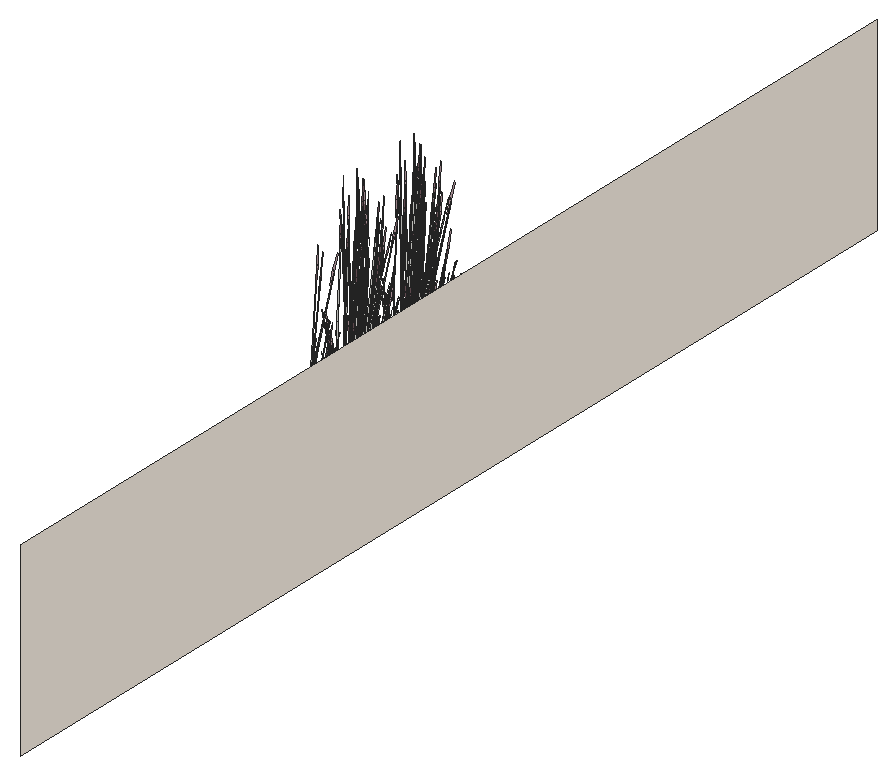
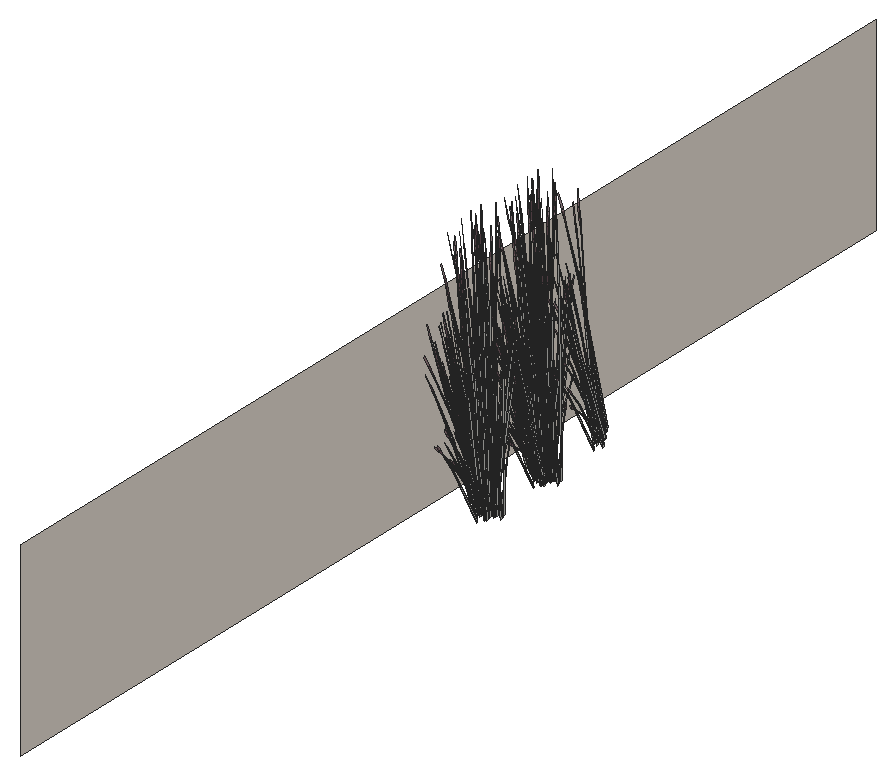
# SketchUp Ruby script. Lengths in inches.
U = 1.inch
M = Sketchup.active_model
def pt(a) = Geom::Point3d.new(a.map { |v| v * U })
def face(e, loops, mat)
  f = e.add_face(loops[0].map { |a| pt(a) })
  loops[1..].each { |l| e.add_face(l.map { |a| pt(a) }).erase! }
  f.material = f.back_material = mat if mat
  f
end
# faces: each face lists its corners as indices into pts; further lists are holes
def faces(e, pts, list, mat = nil) = list.each { |f| face(e, (f[0].is_a?(Array) ? f : [f]).map { |l| l.map { |i| pts[i] } }, mat) }
# xy, xz, yz: faces in a plane at the given z, y or x. An outline is a flat list of corners, or four numbers for a rectangle; further outlines are holes
def ring(l) = l.size == 4 ? [[l[0], l[1]], [l[2], l[1]], [l[2], l[3]], [l[0], l[3]]] : l.each_slice(2).to_a
def flat(e, list, mat, &to3) = list.each { |f| face(e, (f[0].is_a?(Array) ? f : [f]).map { |l| ring(l).map { |u, v| to3.(u, v) } }, mat) }
def xy(e, z, list, mat = nil) = flat(e, list, mat) { |x, y| [x, y, z] }
def xz(e, y, list, mat = nil) = flat(e, list, mat) { |x, z| [x, y, z] }
def yz(e, x, list, mat = nil) = flat(e, list, mat) { |y, z| [x, y, z] }
def lines(e, pts, list) = list.each { |a, b| e.add_line(pt(pts[a]), pt(pts[b])) }
# prism: a flat outline (further loops are holes) pulled along v
def prism(e, loops, v, mat = nil)
  f = face(e, loops, mat); d = Geom::Vector3d.new(v.map { |x| x * U })
  f.pushpull(f.normal.samedirection?(d) ? d.length : -d.length)
end
def box(e, o, s, mat = nil) = prism(e, [[o, [o[0] + s[0], o[1], o[2]], [o[0] + s[0], o[1] + s[1], o[2]], [o[0], o[1] + s[1], o[2]]]], [0, 0, s[2]], mat)
def at(x, y, z, deg = 0) = Geom::Transformation.translation(pt([x, y, z])) * Geom::Transformation.rotation(ORIGIN, Z_AXIS, deg.degrees)
def axes(o, x, y, z) = Geom::Transformation.new([*x, 0, *y, 0, *z, 0, *pt(o).to_a, 1])
def part(name) = M.definitions.add(name)
# library, detail: a bought-in or finely detailed component or shape, given as its bounding box
def library(name, o, s) = part(name).tap { |d| box(d.entities, o, s) }
def detail(e, o, s) = box(e.add_group.entities, o, s)
def put(e, d, t, mat = nil) = e.add_instance(d, t).tap { |i| i.material = mat if mat }
def group(e, t, mat = nil) = e.add_group.tap { |g| g.transformation = t; g.material = mat if mat }.entities
root = M.entities
M.materials.add("C01_Vanilla_Cream").color = [255, 246, 235]
M.materials.add("LightPink_Translucent").color = [144, 107, 117]
M.materials["LightPink_Translucent"].alpha = 0.75
c1 = part("blade")
p = [[2.15,0.21,22],[0,0.17,0],[0.09,0.45,0],[2.18,0.31,22],[2.29,0.31,22],[0.38,0.45,0],
  [2.48,0.24,33],[2.49,0.24,33],[2.48,0.22,33]]
faces(c1.entities,p,[[0,1,2,3],[4,5,2,3],[6,3,4,7],[8,0,3,6]])
c2 = part("seeds")
p = [[0.3,-0.1,1.38],[-0.01,-0.03,1.59],[-0.01,-0.03,0.03],[0.14,-0.07,-0.07],[0.29,-0.03,3],[0.15,0.01,3.11]]
faces(c2.entities,p,[[0,1,2,3],[1,0,4,5]],"LightPink_Translucent")
c3 = part("blade with seeds")
put(c3.entities,c1,at(0,0,0))
put(c3.entities,c2,axes([2.4,0.25,30.99],[1.5799,-0.05474,1.17369],[-0.12525,1.92788,0.29478],[-0.07173,-0.02425,1.56792]))
yz(root,354,[[30,654,234,690]],"C01_Vanilla_Cream")
put(root,c3,axes([342.72,109.8,658.14],[-0.07631,-0.33368,0.29039],[0.43626,-0.08811,-0.3749],[0.11718,0.09562,0.71734]))
put(root,c3,axes([344.36,108.77,655.65],[0,0.41426,-0.40713],[-0.55282,0,0],[0,0.09435,1.29153]))
put(root,c3,axes([342.97,108.82,657.18],[-0.18354,-0.07137,1.40529],[0.37983,-0.29943,0.11363],[0.23673,0.13508,0.60075]))
put(root,c3,axes([343.01,107.88,657.67],[-0.42697,-0.21524,1.13392],[0.45084,-0.33512,0.48925],[0.13776,0.20196,1.09604]))
put(root,c3,axes([343.65,109.63,656.27],[-0.27821,-0.11912,0.94186],[0.35924,-0.12103,0.69201],[0.09689,0.10252,0.20745]))
put(root,c3,axes([342.68,109.97,658.13],[0.29444,-0.35459,-0.09971],[0.4264,0.20428,-0.55346],[0.14822,0.10018,0.84097]))
put(root,c3,axes([342.29,110.27,657.86],[0.00146,-0.05015,1.45454],[0.42344,-0.22127,-0.13744],[0.14708,0.07898,0.2574]))
put(root,c3,axes([343.73,110.07,655.22],[0.036,-0.05981,1.44601],[0.45322,-0.17614,-0.2209],[0.1374,0.09116,0.2463]))
put(root,c3,axes([343.13,108.72,655.72],[0.18118,0.37929,-0.56754],[-0.52191,0.1366,-0.14895],[0.02003,0.12844,1.25274]))
put(root,c3,axes([343.03,109.8,657.84],[0.48758,-0.09847,-0.41901],[0.08529,0.37293,-0.32456],[0.13096,0.10687,0.80174]))
put(root,c3,axes([341.67,109.85,658.14],[0.14896,-0.31857,0.29039],[0.4346,0.09292,-0.3749],[0.03985,0.12826,0.71734]))
put(root,c3,axes([343.7,110.17,656.1875],[-0.31686,-0.01299,0.86149],[0.20925,-0.27594,0.47565],[0.12517,0.09804,0.67577]))
put(root,c3,axes([342.79,110.1,657.88],[-0.22457,0.26316,0.05273],[-0.3198,-0.15321,0.41509],[0.10339,0.08437,0.63295]))
put(root,c3,axes([342.26,110.99,658.63],[0.34145,-0.23766,-0.0532],[0.31287,0.26029,-0.24121],[0.02203,0.07375,0.7956]))
put(root,c3,axes([342.88,110.03,657.88],[-0.49145,0.09507,0.39362],[-0.08529,-0.37293,0.32456],[0.11558,0.10991,0.8145]))
put(root,c3,axes([342.66,109.51,656.125],[0.00872,-0.13732,1.17261],[0.41669,-0.15339,-0.25218],[0.12863,0.16436,0.50135]))
put(root,c3,axes([341.53,109.99,658.13],[0.48353,-0.19287,-0.09971],[0.23761,0.34232,-0.55346],[0.0638,0.14425,0.84097]))
put(root,c3,axes([341.94,109.97,657.84],[0.48573,0.10385,-0.41901],[-0.16649,0.35605,-0.32456],[0.04454,0.14335,0.80174]))
put(root,c3,axes([342.22,109.23,657.18],[-0.11295,-0.13301,1.40529],[0.52192,-0.11198,0.11363],[0.11796,0.20881,0.60075]))
put(root,c3,axes([341.77,109.9,658.08],[0.23583,0.33684,-0.58257],[-0.48546,0.18772,0.0703],[0.05515,0.16275,0.8241]))
put(root,c3,axes([341.41,110.75,657.87],[0.06263,0.06671,1.43454],[0.50546,0.02621,-0.22687],[0.05083,0.14712,0.11505]))
put(root,c3,axes([343.01,120.83,656.125],[-0.14045,0.08385,1.17261],[-0.42064,-0.14676,-0.25218],[0.07797,-0.18252,0.50135]))
put(root,c3,axes([343.35,121.45,658.08],[0.01286,-0.38319,-0.58257],[0.54141,0.02574,0.0703],[0.05714,-0.16234,0.8241]))
put(root,c3,axes([344.11,120.86,657.87],[-0.00477,-0.08245,1.43454],[-0.40285,-0.23829,-0.22687],[0.06228,-0.14445,0.11505]))
put(root,c3,axes([342.74,121.26,657.18],[-0.092,0.14239,1.40529],[-0.38596,-0.29467,0.11363],[0.17411,-0.18366,0.60075]))
put(root,c3,axes([344,120.56,657.86],[-0.05018,0.03164,1.45454],[-0.49165,-0.10676,-0.13744],[-0.0178,-0.13809,0.2574]))
put(root,c3,axes([342.49,120.17,656.27],[0.06339,0.24157,0.94186],[-0.35163,-0.13379,0.69201],[0.03784,-0.12369,0.20745]))
put(root,c3,axes([343.24,121.33,657.84],[-0.35372,-0.27835,-0.41901],[0.37366,-0.24377,-0.32456],[0.05382,-0.14142,0.80174]))
put(root,c3,axes([342.47,120.91,657.88],[0.48688,0.1083,0.39362],[-0.16649,0.35605,0.32456],[-0.02926,-0.14002,0.8145]))
put(root,c3,axes([343.61,121.47,658.13],[-0.54305,-0.02053,-0.09971],[0.01484,-0.38862,-0.55346],[0.03772,-0.14967,0.84097]))
put(root,c3,axes([343.57,121.22,657.71],[0.33433,-0.21811,-0.29039],[0.31649,0.24905,0.3749],[0.04815,-0.12654,0.71734]))
put(root,c3,axes([342.6,120.89,657.88],[0.36409,-0.14079,0.05273],[0.17821,0.25674,0.41509],[-0.03516,-0.11317,0.63295]))
put(root,c3,axes([343.99,121.09,655.22],[-0.07396,-0.03263,1.44601],[-0.18997,-0.3646,-0.2209],[0.12815,-0.09894,0.2463]))
put(root,c3,axes([343.57,121.31,657.88],[0.35185,0.28265,0.39362],[-0.37366,0.24377,0.32456],[0.0649,-0.13261,0.8145]))
put(root,c3,axes([343.7,121.34,657.88],[0.40605,0.0193,0.05273],[-0.01113,0.29147,0.41509],[0.04249,-0.11165,0.63295]))
put(root,c3,axes([343.4,121.53,658.14],[-0.33433,0.21811,0.29039],[-0.31649,-0.24905,-0.3749],[0.04815,-0.12654,0.71734]))
put(root,c3,axes([343.99,122.12,658.08],[0.2581,-0.32687,-0.58257],[0.45228,0.2323,0.0703],[0.15411,-0.11843,0.8241]))
put(root,c3,axes([341.2,121.17,655.95],[-0.30893,-0.41511,0],[0.51685,-0.2315,-0.42318],[0.11772,-0.05273,1.34243]))
put(root,c3,axes([343.98,121.97,657.84],[-0.12693,-0.37826,-0.41901],[0.48071,-0.06617,-0.32456],[0.13776,-0.1016,0.80174]))
put(root,c3,axes([344.2,122.24,658.13],[-0.45707,-0.22842,-0.09971],[0.26332,-0.3308,-0.55346],[0.12913,-0.11499,0.84097]))
put(root,c3,axes([341.62,121.1,655.65],[0.46245,-0.20713,-0.40713],[0.27641,0.37142,0],[0.10533,-0.04718,1.29153]))
put(root,c3,axes([344.36,121.82,656.125],[-0.17652,-0.01227,1.17261],[-0.18084,-0.32916,-0.25218],[0.21685,-0.09312,0.50135]))
put(root,c3,axes([345.33,122.14,657.86],[-0.06454,-0.00315,1.45454],[-0.268,-0.33712,-0.13744],[0.10763,-0.11085,0.2574]))
put(root,c3,axes([342.17,121.95,655.6875],[0.33282,-0.31137,-0.51129],[0.41344,0.28235,-0.13419],[0.13336,-0.07767,1.12859]))
put(root,c3,axes([344.57,121.22,656.27],[-0.16458,0.21088,0.94186],[-0.14146,-0.28332,0.69201],[0.13593,-0.07099,0.20745]))
put(root,c3,axes([344.33,122.01,657.71],[0.43011,-0.0592,-0.29039],[0.11357,0.33844,0.3749],[0.12326,-0.0909,0.71734]))
put(root,c3,axes([341.81,122.31,656.1875],[-0.05758,-0.4727,-0.23858],[0.59969,-0.02858,-0.41002],[0.1056,-0.06296,1.3096]))
put(root,c3,axes([343.98,122.21,658.14],[-0.43011,0.0592,0.29039],[-0.11357,-0.33844,-0.3749],[0.12326,-0.0909,0.71734]))
put(root,c3,axes([341.73,121.27,655.66],[0.46099,0.1025,-0.25402],[-0.11607,0.36097,0.25402],[0.09293,-0.04163,1.13959]))
put(root,c3,axes([344.37,122.15,657.88],[0.33921,0.17422,0.05273],[-0.19749,0.2481,0.41509],[0.10876,-0.08021,0.63295]))
put(root,c3,axes([344.27,122.08,657.88],[0.12254,0.38127,0.39362],[-0.48071,0.06617,0.32456],[0.14168,-0.08967,0.8145]))
put(root,c3,axes([345.57,122.54,657.87],[0.06857,-0.0631,1.43454],[-0.08776,-0.38707,-0.22687],[0.17204,-0.07339,0.11505]))
put(root,c3,axes([341.88,122.69,656],[0.55674,0.20078,0.19733],[-0.26794,0.4172,0.41002],[0,-0.09617,1.31645]))
put(root,c3,axes([341.7,122.41,656.23],[-0.53657,0.02557,0.36686],[-0.04852,-0.4245,-0.17656],[0.09606,-0.04302,1.17788]))
put(root,c3,axes([344.22,123.13,658.13],[-0.24861,-0.37512,-0.09971],[0.44125,-0.18434,-0.55346],[0.18594,-0.04949,0.84097]))
put(root,c3,axes([344.2,122.81,657.84],[0.13386,-0.37682,-0.41901],[0.45895,0.12916,-0.32456],[0.18478,-0.03455,0.80174]))
put(root,c3,axes([343.47,121.27,655.95],[0.30893,-0.41511,0],[0.51685,0.2315,-0.42318],[0.11772,0.05273,1.34243]))
put(root,c3,axes([344.6875,122.91,655.625],[-0.31825,0.04971,1.16098],[-0.05066,-0.39572,0.06645],[0.2229,-0.0599,0.66064]))
put(root,c3,axes([345.27,122.5625,655.85],[-0.30634,-0.2649,-0.0532],[0.33551,-0.24272,-0.24121],[0.09507,-0.01709,0.7956]))
put(root,c3,axes([342.46,122.6,655.81],[0,-0.47933,0],[0.61786,0,0],[0,0,1.47154]))
put(root,c3,axes([343.21,121.49,656.03],[-0.46245,-0.20713,0.40713],[0.27641,-0.37142,0],[0.10533,0.04718,1.29153]))
put(root,c3,axes([344.11,122.94,658.08],[0.43419,-0.18296,-0.58257],[0.24197,0.37661,0.0703],[0.20979,-0.04278,0.8241]))
put(root,c3,axes([342.17,122.3,655.9375],[-0.40969,0.37595,0.37519],[-0.48673,-0.33186,0.14723],[0.09877,-0.03752,1.30262]))
put(root,c3,axes([341.45,121.68,656.03],[-0.14274,0.41171,0.14467],[-0.52234,-0.11651,0.28771],[0.09023,-0.00201,1.31534]))
put(root,c3,axes([344.05,123.02,658.14],[-0.41064,-0.11557,0.29039],[0.11977,-0.33716,-0.3749],[0.16533,-0.03092,0.71734]))
put(root,c3,axes([341.24,122.01,655.31],[-0.48636,0.16585,1.05721],[-0.1548,-0.47588,0.41079],[0.29865,0.00792,1.20246]))
put(root,c3,axes([342.54,122.13,656.15],[0.09532,-0.36971,0.11873],[0.46572,0.06418,-0.33905],[0.08476,0.03796,1.0393]))
put(root,c3,axes([345.04,122.66,655.22],[-0.02582,-0.06289,1.44601],[0.17911,-0.36789,-0.2209],[0.18067,-0.00529,0.2463]))
put(root,c3,axes([342.35,122.23,656.23],[-0.29683,-0.34771,0.36686],[0.44961,-0.24485,-0.17656],[0.09606,0.04302,1.17788]))
put(root,c3,axes([342.5,122.25,656.1875],[0.49889,-0.27503,-0.23858],[0.33175,0.38862,-0.41002],[0.12309,0.03947,1.3096]))
put(root,c3,axes([344.48,122.98,657.71],[0.41064,0.11557,-0.29039],[-0.11977,0.33716,0.3749],[0.16533,-0.03092,0.71734]))
put(root,c3,axes([343.75,121.52,655.65],[0.46245,0.20713,-0.40713],[-0.27641,0.37142,0],[0.10533,0.04718,1.29153]))
put(root,c3,axes([342.88,122.7,655.81],[0.55282,0,0],[0,0.42888,0],[0,0,1.46294]))
put(root,c3,axes([343.03,121.7,656.03],[-0.53096,0.10995,0.14467],[-0.13111,-0.40919,0.28771],[0.04735,0.05962,1.31534]))
put(root,c3,axes([343.36,122.5625,657.18],[-0.20495,0.00938,1.40529],[0.13596,-0.40664,0.11363],[0.29207,0.02515,0.60075]))
put(root,c3,axes([343.625,121.68,655.66],[0.11607,0.36097,-0.25402],[-0.46099,0.1025,0.25402],[0.09293,0.04163,1.13959]))
put(root,c3,axes([344.42,123.12,657.88],[0.18148,0.28246,0.05273],[-0.33093,0.13825,0.41509],[0.14588,-0.02728,0.63295]))
put(root,c3,axes([342.7,122.49,655.95],[-0.62452,-0.08728,0.40343],[0.1271,-0.49295,0.15831],[0.09127,0.0476,1.40067]))
put(root,c3,axes([344.39,123.02,657.88],[-0.1396,0.37772,0.39362],[-0.45895,-0.12916,0.32456],[0.18049,-0.0227,0.8145]))
put(root,c3,axes([342.8,123.65,655.79],[0.51876,-0.14056,-0.15742],[0.18228,0.40489,0.00007],[0.05726,-0.01554,1.42596]))
put(root,c3,axes([342.87,122.89,655.82],[0.34492,0.26758,0],[-0.34492,0.26758,0],[0,0,1.38798]))
put(root,c3,axes([343.8,122.77,656.03],[-0.38822,-0.30175,0.14467],[0.39123,-0.29268,0.28771],[-0.04288,0.06162,1.31534]))
put(root,c3,axes([343.08,122.32,655.6875],[0.514,0.06792,-0.51129],[-0.10846,0.41895,-0.13419],[0.15339,0.05076,1.12859]))
put(root,c3,axes([345.35,123.05,656.27],[-0.30529,0.06839,0.94186],[0.1437,-0.28265,0.69201],[0.16196,0.01934,0.20745]))
put(root,c3,axes([342.86,122.58,656.23],[0.23974,-0.37328,0.36686],[0.49814,0.17965,-0.17656],[0,0.08605,1.17788]))
put(root,c3,axes([345.21,124.24,657.86],[-0.04468,-0.03627,1.45454],[0.09773,-0.38875,-0.13744],[0.17599,-0.02484,0.2574]))
put(root,c3,axes([342.77,122.79,655.88],[0,0.4791,-0.04622],[-0.61786,0,0],[0,0.01506,1.47081]))
put(root,c3,axes([342.8125,122.45,655.8125],[0.29683,0.34771,-0.36686],[-0.44961,0.24485,0.17656],[0.09606,0.04302,1.17788]))
put(root,c3,axes([344.82,123.92,657.22],[-0.09457,-0.34824,-0.02863],[0.44699,-0.08006,-0.12982],[0.09334,0.02208,0.42819]))
put(root,c3,axes([343.66,123.91,658.13],[0.02646,-0.4213,-0.09971],[0.50094,0.01152,-0.55346],[0.19293,0.02926,0.84097]))
put(root,c3,axes([344.12,122.78,656.03],[0,-0.41426,0.40713],[0.55282,0,0],[0,0.09435,1.29153]))
put(root,c3,axes([343.07,122.66,656.15],[0.46037,-0.12081,0.11873],[0.16122,0.34498,-0.33905],[0,0.07592,1.0393]))
put(root,c3,axes([343.59,123.74,658.14],[-0.28114,-0.25937,0.29039],[0.32102,-0.24553,-0.3749],[0.16311,0.03736,0.71734]))
put(root,c3,axes([344.78,123.5,656.125],[-0.119,-0.10189,1.17261],[0.15483,-0.33705,-0.25218],[0.24077,0.04566,0.50135]))
put(root,c3,axes([342.65,123.87,655.81],[0.49814,0.18599,0],[-0.23974,0.38645,0],[0,0,1.43462]))
put(root,c3,axes([344.1,123.66,657.87],[0.106,-0.00701,1.43454],[0.29074,-0.32184,-0.22687],[0.18854,0.04248,0.11505]))
put(root,c3,axes([343.6875,123.71,658.08],[0.49394,0.00997,-0.58257],[-0.03317,0.42002,0.0703],[0.20925,0.04433,0.8241]))
put(root,c3,axes([342.47,123.72,655.88],[0.21483,0.47591,-0.0493],[-0.61383,0.16676,0],[0.0075,0.01662,1.41182]))
put(root,c3,axes([344.49,122.85,655.95],[0.61786,0,0],[0,0.463,-0.42318],[0,0.10545,1.34243]))
put(root,c3,axes([344.25,123.09,655.8],[-0.61756,-0.00331,-0.04081],[0,-0.463,0.40953],[-0.01941,0.1054,1.29849]))
put(root,c3,axes([342.91,122.6875,656.1875],[0.55647,0.19766,-0.23858],[-0.26794,0.4172,-0.41002],[0.01749,0.10243,1.3096]))
put(root,c3,axes([343.98,123.88,657.71],[0.28114,0.25937,-0.29039],[-0.32102,0.24553,0.3749],[0.16311,0.03736,0.71734]))
put(root,c3,axes([344.12,123.16,655.66],[-0.34492,0.25847,-0.25402],[-0.34492,-0.25847,0.25402],[0,0.08325,1.13959]))
put(root,c3,axes([343.84,123.98,657.88],[-0.02488,0.31501,0.05273],[-0.3757,-0.00864,0.41509],[0.14392,0.03296,0.63295]))
put(root,c3,axes([342.85,123,655.8125],[-0.23974,0.37328,-0.36686],[-0.49814,-0.17965,0.17656],[0,0.08605,1.17788]))
put(root,c3,axes([343.875,123.88,657.88],[-0.36434,0.27297,0.39362],[-0.31422,-0.28988,0.32456],[0.17094,0.05035,0.8145]))
put(root,c3,axes([342.72,124.19,658.14],[-0.07631,-0.33368,0.29039],[0.43626,-0.08811,-0.3749],[0.11718,0.09562,0.71734]))
put(root,c3,axes([344.36,123.17,655.65],[0,0.41426,-0.40713],[-0.55282,0,0],[0,0.09435,1.29153]))
put(root,c3,axes([342.97,123.21,657.18],[-0.18354,-0.07137,1.40529],[0.37983,-0.29943,0.11363],[0.23673,0.13508,0.60075]))
put(root,c3,axes([343.01,122.28,657.67],[-0.42697,-0.21524,1.13392],[0.45084,-0.33512,0.48925],[0.13776,0.20196,1.09604]))
put(root,c3,axes([343.65,124.03,656.27],[-0.27821,-0.11912,0.94186],[0.35924,-0.12103,0.69201],[0.09689,0.10252,0.20745]))
put(root,c3,axes([342.68,124.37,658.13],[0.29444,-0.35459,-0.09971],[0.4264,0.20428,-0.55346],[0.14822,0.10018,0.84097]))
put(root,c3,axes([342.29,124.66,657.86],[0.00146,-0.05015,1.45454],[0.42344,-0.22127,-0.13744],[0.14708,0.07898,0.2574]))
put(root,c3,axes([343.73,124.47,655.22],[0.036,-0.05981,1.44601],[0.45322,-0.17614,-0.2209],[0.1374,0.09116,0.2463]))
put(root,c3,axes([343.13,123.11,655.72],[0.18118,0.37929,-0.56754],[-0.52191,0.1366,-0.14895],[0.02003,0.12844,1.25274]))
put(root,c3,axes([343.03,124.19,657.84],[0.48758,-0.09847,-0.41901],[0.08529,0.37293,-0.32456],[0.13096,0.10687,0.80174]))
put(root,c3,axes([341.67,124.25,658.14],[0.14896,-0.31857,0.29039],[0.4346,0.09292,-0.3749],[0.03985,0.12826,0.71734]))
put(root,c3,axes([343.7,124.57,656.1875],[-0.31686,-0.01299,0.86149],[0.20925,-0.27594,0.47565],[0.12517,0.09804,0.67577]))
put(root,c3,axes([342.79,124.5,657.88],[-0.22457,0.26316,0.05273],[-0.3198,-0.15321,0.41509],[0.10339,0.08437,0.63295]))
put(root,c3,axes([342.26,125.38,658.63],[0.34145,-0.23766,-0.0532],[0.31287,0.26029,-0.24121],[0.02203,0.07375,0.7956]))
put(root,c3,axes([342.88,124.42,657.88],[-0.49145,0.09507,0.39362],[-0.08529,-0.37293,0.32456],[0.11558,0.10991,0.8145]))
put(root,c3,axes([342.66,123.9,656.125],[0.00872,-0.13732,1.17261],[0.41669,-0.15339,-0.25218],[0.12863,0.16436,0.50135]))
put(root,c3,axes([341.53,124.38,658.13],[0.48353,-0.19287,-0.09971],[0.23761,0.34232,-0.55346],[0.0638,0.14425,0.84097]))
put(root,c3,axes([341.94,124.36,657.84],[0.48573,0.10385,-0.41901],[-0.16649,0.35605,-0.32456],[0.04454,0.14335,0.80174]))
put(root,c3,axes([342.22,123.63,657.18],[-0.11295,-0.13301,1.40529],[0.52192,-0.11198,0.11363],[0.11796,0.20881,0.60075]))
put(root,c3,axes([341.77,124.3,658.08],[0.23583,0.33684,-0.58257],[-0.48546,0.18772,0.0703],[0.05515,0.16275,0.8241]))
put(root,c3,axes([341.41,125.15,657.87],[0.06263,0.06671,1.43454],[0.50546,0.02621,-0.22687],[0.05083,0.14712,0.11505]))
put(root,c3,axes([343.01,134.32,656.125],[-0.14045,0.08385,1.17261],[-0.42064,-0.14676,-0.25218],[0.07797,-0.18252,0.50135]))
put(root,c3,axes([343.35,134.94,658.08],[0.01286,-0.38319,-0.58257],[0.54141,0.02574,0.0703],[0.05714,-0.16234,0.8241]))
put(root,c3,axes([344.11,134.35,657.87],[-0.00477,-0.08245,1.43454],[-0.40285,-0.23829,-0.22687],[0.06228,-0.14445,0.11505]))
put(root,c3,axes([342.74,134.75,657.18],[-0.092,0.14239,1.40529],[-0.38596,-0.29467,0.11363],[0.17411,-0.18366,0.60075]))
put(root,c3,axes([344,134.05,657.86],[-0.05018,0.03164,1.45454],[-0.49165,-0.10676,-0.13744],[-0.0178,-0.13809,0.2574]))
put(root,c3,axes([342.49,133.66,656.27],[0.06339,0.24157,0.94186],[-0.35163,-0.13379,0.69201],[0.03784,-0.12369,0.20745]))
put(root,c3,axes([343.24,134.82,657.84],[-0.35372,-0.27835,-0.41901],[0.37366,-0.24377,-0.32456],[0.05382,-0.14142,0.80174]))
put(root,c3,axes([342.47,134.4,657.88],[0.48688,0.1083,0.39362],[-0.16649,0.35605,0.32456],[-0.02926,-0.14002,0.8145]))
put(root,c3,axes([343.61,134.96,658.13],[-0.54305,-0.02053,-0.09971],[0.01484,-0.38862,-0.55346],[0.03772,-0.14967,0.84097]))
put(root,c3,axes([343.57,134.71,657.71],[0.33433,-0.21811,-0.29039],[0.31649,0.24905,0.3749],[0.04815,-0.12654,0.71734]))
put(root,c3,axes([342.6,134.375,657.88],[0.36409,-0.14079,0.05273],[0.17821,0.25674,0.41509],[-0.03516,-0.11317,0.63295]))
put(root,c3,axes([343.99,134.58,655.22],[-0.07396,-0.03263,1.44601],[-0.18997,-0.3646,-0.2209],[0.12815,-0.09894,0.2463]))
put(root,c3,axes([343.57,134.8,657.88],[0.35185,0.28265,0.39362],[-0.37366,0.24377,0.32456],[0.0649,-0.13261,0.8145]))
put(root,c3,axes([343.7,134.83,657.88],[0.40605,0.0193,0.05273],[-0.01113,0.29147,0.41509],[0.04249,-0.11165,0.63295]))
put(root,c3,axes([343.4,135.02,658.14],[-0.33433,0.21811,0.29039],[-0.31649,-0.24905,-0.3749],[0.04815,-0.12654,0.71734]))
put(root,c3,axes([343.99,135.61,658.08],[0.2581,-0.32687,-0.58257],[0.45228,0.2323,0.0703],[0.15411,-0.11843,0.8241]))
put(root,c3,axes([341.2,134.66,655.95],[-0.30893,-0.41511,0],[0.51685,-0.2315,-0.42318],[0.11772,-0.05273,1.34243]))
put(root,c3,axes([343.98,135.46,657.84],[-0.12693,-0.37826,-0.41901],[0.48071,-0.06617,-0.32456],[0.13776,-0.1016,0.80174]))
put(root,c3,axes([344.2,135.73,658.13],[-0.45707,-0.22842,-0.09971],[0.26332,-0.3308,-0.55346],[0.12913,-0.11499,0.84097]))
put(root,c3,axes([341.62,134.59,655.65],[0.46245,-0.20713,-0.40713],[0.27641,0.37142,0],[0.10533,-0.04718,1.29153]))
put(root,c3,axes([344.36,135.3125,656.125],[-0.17652,-0.01227,1.17261],[-0.18084,-0.32916,-0.25218],[0.21685,-0.09312,0.50135]))
put(root,c3,axes([345.33,135.63,657.86],[-0.06454,-0.00315,1.45454],[-0.268,-0.33712,-0.13744],[0.10763,-0.11085,0.2574]))
put(root,c3,axes([342.17,135.44,655.6875],[0.33282,-0.31137,-0.51129],[0.41344,0.28235,-0.13419],[0.13336,-0.07767,1.12859]))
put(root,c3,axes([344.57,134.71,656.27],[-0.16458,0.21088,0.94186],[-0.14146,-0.28332,0.69201],[0.13593,-0.07099,0.20745]))
put(root,c3,axes([344.33,135.5,657.71],[0.43011,-0.0592,-0.29039],[0.11357,0.33844,0.3749],[0.12326,-0.0909,0.71734]))
put(root,c3,axes([341.81,135.81,656.1875],[-0.05758,-0.4727,-0.23858],[0.59969,-0.02858,-0.41002],[0.1056,-0.06296,1.3096]))
put(root,c3,axes([343.98,135.7,658.14],[-0.43011,0.0592,0.29039],[-0.11357,-0.33844,-0.3749],[0.12326,-0.0909,0.71734]))
put(root,c3,axes([341.73,134.76,655.66],[0.46099,0.1025,-0.25402],[-0.11607,0.36097,0.25402],[0.09293,-0.04163,1.13959]))
put(root,c3,axes([344.37,135.64,657.88],[0.33921,0.17422,0.05273],[-0.19749,0.2481,0.41509],[0.10876,-0.08021,0.63295]))
put(root,c3,axes([344.27,135.57,657.88],[0.12254,0.38127,0.39362],[-0.48071,0.06617,0.32456],[0.14168,-0.08967,0.8145]))
put(root,c3,axes([345.57,136.03,657.87],[0.06857,-0.0631,1.43454],[-0.08776,-0.38707,-0.22687],[0.17204,-0.07339,0.11505]))
put(root,c3,axes([341.88,136.18,656],[0.55674,0.20078,0.19733],[-0.26794,0.4172,0.41002],[0,-0.09617,1.31645]))
put(root,c3,axes([341.7,135.9,656.23],[-0.53657,0.02557,0.36686],[-0.04852,-0.4245,-0.17656],[0.09606,-0.04302,1.17788]))
put(root,c3,axes([344.22,136.62,658.13],[-0.24861,-0.37512,-0.09971],[0.44125,-0.18434,-0.55346],[0.18594,-0.04949,0.84097]))
put(root,c3,axes([344.2,136.3,657.84],[0.13386,-0.37682,-0.41901],[0.45895,0.12916,-0.32456],[0.18478,-0.03455,0.80174]))
put(root,c3,axes([343.47,134.76,655.95],[0.30893,-0.41511,0],[0.51685,0.2315,-0.42318],[0.11772,0.05273,1.34243]))
put(root,c3,axes([344.6875,136.4,655.625],[-0.31825,0.04971,1.16098],[-0.05066,-0.39572,0.06645],[0.2229,-0.0599,0.66064]))
put(root,c3,axes([345.27,136.05,655.85],[-0.30634,-0.2649,-0.0532],[0.33551,-0.24272,-0.24121],[0.09507,-0.01709,0.7956]))
put(root,c3,axes([342.46,136.09,655.81],[0,-0.47933,0],[0.61786,0,0],[0,0,1.47154]))
put(root,c3,axes([343.21,134.98,656.03],[-0.46245,-0.20713,0.40713],[0.27641,-0.37142,0],[0.10533,0.04718,1.29153]))
put(root,c3,axes([344.11,136.44,658.08],[0.43419,-0.18296,-0.58257],[0.24197,0.37661,0.0703],[0.20979,-0.04278,0.8241]))
put(root,c3,axes([342.17,135.79,655.9375],[-0.40969,0.37595,0.37519],[-0.48673,-0.33186,0.14723],[0.09877,-0.03752,1.30262]))
put(root,c3,axes([341.45,135.17,656.03],[-0.14274,0.41171,0.14467],[-0.52234,-0.11651,0.28771],[0.09023,-0.00201,1.31534]))
put(root,c3,axes([344.05,136.51,658.14],[-0.41064,-0.11557,0.29039],[0.11977,-0.33716,-0.3749],[0.16533,-0.03092,0.71734]))
put(root,c3,axes([341.24,135.5,655.31],[-0.48636,0.16585,1.05721],[-0.1548,-0.47588,0.41079],[0.29865,0.00792,1.20246]))
put(root,c3,axes([342.54,135.625,656.15],[0.09532,-0.36971,0.11873],[0.46572,0.06418,-0.33905],[0.08476,0.03796,1.0393]))
put(root,c3,axes([345.04,136.15,655.22],[-0.02582,-0.06289,1.44601],[0.17911,-0.36789,-0.2209],[0.18067,-0.00529,0.2463]))
put(root,c3,axes([342.35,135.72,656.23],[-0.29683,-0.34771,0.36686],[0.44961,-0.24485,-0.17656],[0.09606,0.04302,1.17788]))
put(root,c3,axes([342.5,135.74,656.1875],[0.49889,-0.27503,-0.23858],[0.33175,0.38862,-0.41002],[0.12309,0.03947,1.3096]))
put(root,c3,axes([344.48,136.47,657.71],[0.41064,0.11557,-0.29039],[-0.11977,0.33716,0.3749],[0.16533,-0.03092,0.71734]))
put(root,c3,axes([343.75,135.01,655.65],[0.46245,0.20713,-0.40713],[-0.27641,0.37142,0],[0.10533,0.04718,1.29153]))
put(root,c3,axes([342.88,136.2,655.81],[0.55282,0,0],[0,0.42888,0],[0,0,1.46294]))
put(root,c3,axes([343.03,135.19,656.03],[-0.53096,0.10995,0.14467],[-0.13111,-0.40919,0.28771],[0.04735,0.05962,1.31534]))
put(root,c3,axes([343.36,136.05,657.18],[-0.20495,0.00938,1.40529],[0.13596,-0.40664,0.11363],[0.29207,0.02515,0.60075]))
put(root,c3,axes([343.625,135.17,655.66],[0.11607,0.36097,-0.25402],[-0.46099,0.1025,0.25402],[0.09293,0.04163,1.13959]))
put(root,c3,axes([344.42,136.61,657.88],[0.18148,0.28246,0.05273],[-0.33093,0.13825,0.41509],[0.14588,-0.02728,0.63295]))
put(root,c3,axes([342.7,135.98,655.95],[-0.62452,-0.08728,0.40343],[0.1271,-0.49295,0.15831],[0.09127,0.0476,1.40067]))
put(root,c3,axes([344.39,136.51,657.88],[-0.1396,0.37772,0.39362],[-0.45895,-0.12916,0.32456],[0.18049,-0.0227,0.8145]))
put(root,c3,axes([342.8,137.14,655.79],[0.51876,-0.14056,-0.15742],[0.18228,0.40489,0.00007],[0.05726,-0.01554,1.42596]))
put(root,c3,axes([342.87,136.38,655.82],[0.34492,0.26758,0],[-0.34492,0.26758,0],[0,0,1.38798]))
put(root,c3,axes([343.8,136.26,656.03],[-0.38822,-0.30175,0.14467],[0.39123,-0.29268,0.28771],[-0.04288,0.06162,1.31534]))
put(root,c3,axes([343.08,135.81,655.6875],[0.514,0.06792,-0.51129],[-0.10846,0.41895,-0.13419],[0.15339,0.05076,1.12859]))
put(root,c3,axes([345.35,136.54,656.27],[-0.30529,0.06839,0.94186],[0.1437,-0.28265,0.69201],[0.16196,0.01934,0.20745]))
put(root,c3,axes([342.86,136.07,656.23],[0.23974,-0.37328,0.36686],[0.49814,0.17965,-0.17656],[0,0.08605,1.17788]))
put(root,c3,axes([345.21,137.73,657.86],[-0.04468,-0.03627,1.45454],[0.09773,-0.38875,-0.13744],[0.17599,-0.02484,0.2574]))
put(root,c3,axes([342.77,136.28,655.88],[0,0.4791,-0.04622],[-0.61786,0,0],[0,0.01506,1.47081]))
put(root,c3,axes([342.8125,135.94,655.8125],[0.29683,0.34771,-0.36686],[-0.44961,0.24485,0.17656],[0.09606,0.04302,1.17788]))
put(root,c3,axes([344.82,137.41,657.22],[-0.09457,-0.34824,-0.02863],[0.44699,-0.08006,-0.12982],[0.09334,0.02208,0.42819]))
put(root,c3,axes([343.66,137.4,658.13],[0.02646,-0.4213,-0.09971],[0.50094,0.01152,-0.55346],[0.19293,0.02926,0.84097]))
put(root,c3,axes([344.12,136.27,656.03],[0,-0.41426,0.40713],[0.55282,0,0],[0,0.09435,1.29153]))
put(root,c3,axes([343.07,136.15,656.15],[0.46037,-0.12081,0.11873],[0.16122,0.34498,-0.33905],[0,0.07592,1.0393]))
put(root,c3,axes([343.59,137.23,658.14],[-0.28114,-0.25937,0.29039],[0.32102,-0.24553,-0.3749],[0.16311,0.03736,0.71734]))
put(root,c3,axes([344.78,136.99,656.125],[-0.119,-0.10189,1.17261],[0.15483,-0.33705,-0.25218],[0.24077,0.04566,0.50135]))
put(root,c3,axes([342.65,137.36,655.81],[0.49814,0.18599,0],[-0.23974,0.38645,0],[0,0,1.43462]))
put(root,c3,axes([344.1,137.15,657.87],[0.106,-0.00701,1.43454],[0.29074,-0.32184,-0.22687],[0.18854,0.04248,0.11505]))
put(root,c3,axes([343.6875,137.2,658.08],[0.49394,0.00997,-0.58257],[-0.03317,0.42002,0.0703],[0.20925,0.04433,0.8241]))
put(root,c3,axes([342.47,137.21,655.88],[0.21483,0.47591,-0.0493],[-0.61383,0.16676,0],[0.0075,0.01662,1.41182]))
put(root,c3,axes([344.49,136.34,655.95],[0.61786,0,0],[0,0.463,-0.42318],[0,0.10545,1.34243]))
put(root,c3,axes([344.25,136.58,655.8],[-0.61756,-0.00331,-0.04081],[0,-0.463,0.40953],[-0.01941,0.1054,1.29849]))
put(root,c3,axes([342.91,136.18,656.1875],[0.55647,0.19766,-0.23858],[-0.26794,0.4172,-0.41002],[0.01749,0.10243,1.3096]))
put(root,c3,axes([343.98,137.37,657.71],[0.28114,0.25937,-0.29039],[-0.32102,0.24553,0.3749],[0.16311,0.03736,0.71734]))
put(root,c3,axes([344.12,136.65,655.66],[-0.34492,0.25847,-0.25402],[-0.34492,-0.25847,0.25402],[0,0.08325,1.13959]))
put(root,c3,axes([343.84,137.47,657.88],[-0.02488,0.31501,0.05273],[-0.3757,-0.00864,0.41509],[0.14392,0.03296,0.63295]))
put(root,c3,axes([342.85,136.49,655.8125],[-0.23974,0.37328,-0.36686],[-0.49814,-0.17965,0.17656],[0,0.08605,1.17788]))
put(root,c3,axes([343.875,137.37,657.88],[-0.36434,0.27297,0.39362],[-0.31422,-0.28988,0.32456],[0.17094,0.05035,0.8145]))
put(root,c3,axes([342.72,137.69,658.14],[-0.07631,-0.33368,0.29039],[0.43626,-0.08811,-0.3749],[0.11718,0.09562,0.71734]))
put(root,c3,axes([344.36,136.66,655.65],[0,0.41426,-0.40713],[-0.55282,0,0],[0,0.09435,1.29153]))
put(root,c3,axes([342.97,136.71,657.18],[-0.18354,-0.07137,1.40529],[0.37983,-0.29943,0.11363],[0.23673,0.13508,0.60075]))
put(root,c3,axes([343.01,135.77,657.67],[-0.42697,-0.21524,1.13392],[0.45084,-0.33512,0.48925],[0.13776,0.20196,1.09604]))
put(root,c3,axes([343.65,137.52,656.27],[-0.27821,-0.11912,0.94186],[0.35924,-0.12103,0.69201],[0.09689,0.10252,0.20745]))
put(root,c3,axes([342.68,137.86,658.13],[0.29444,-0.35459,-0.09971],[0.4264,0.20428,-0.55346],[0.14822,0.10018,0.84097]))
put(root,c3,axes([342.29,138.15,657.86],[0.00146,-0.05015,1.45454],[0.42344,-0.22127,-0.13744],[0.14708,0.07898,0.2574]))
put(root,c3,axes([343.73,137.96,655.22],[0.036,-0.05981,1.44601],[0.45322,-0.17614,-0.2209],[0.1374,0.09116,0.2463]))
put(root,c3,axes([343.13,136.6,655.72],[0.18118,0.37929,-0.56754],[-0.52191,0.1366,-0.14895],[0.02003,0.12844,1.25274]))
put(root,c3,axes([343.03,137.68,657.84],[0.48758,-0.09847,-0.41901],[0.08529,0.37293,-0.32456],[0.13096,0.10687,0.80174]))
put(root,c3,axes([341.67,137.74,658.14],[0.14896,-0.31857,0.29039],[0.4346,0.09292,-0.3749],[0.03985,0.12826,0.71734]))
put(root,c3,axes([343.7,138.06,656.1875],[-0.31686,-0.01299,0.86149],[0.20925,-0.27594,0.47565],[0.12517,0.09804,0.67577]))
put(root,c3,axes([342.79,137.99,657.88],[-0.22457,0.26316,0.05273],[-0.3198,-0.15321,0.41509],[0.10339,0.08437,0.63295]))
put(root,c3,axes([342.26,138.875,658.63],[0.34145,-0.23766,-0.0532],[0.31287,0.26029,-0.24121],[0.02203,0.07375,0.7956]))
put(root,c3,axes([342.88,137.91,657.88],[-0.49145,0.09507,0.39362],[-0.08529,-0.37293,0.32456],[0.11558,0.10991,0.8145]))
